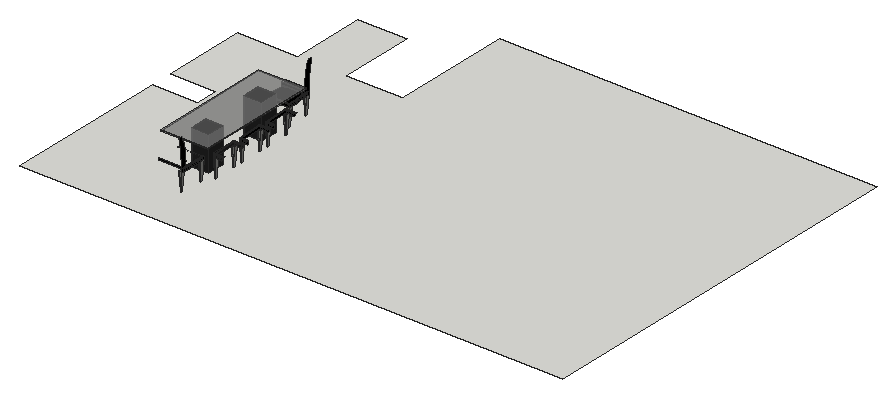
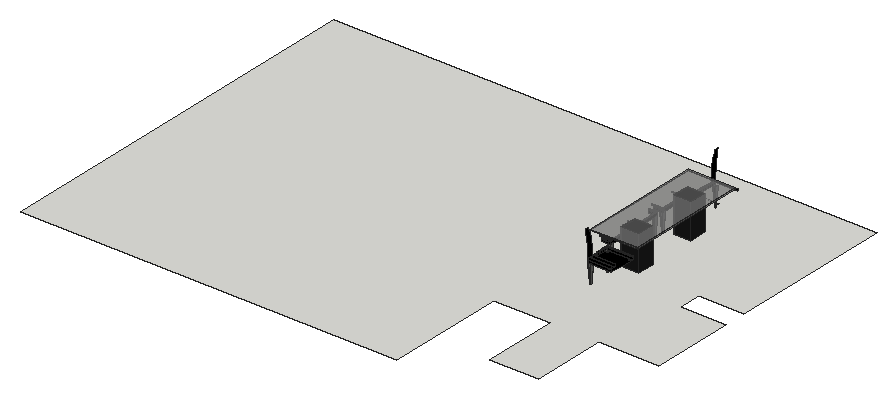
# SketchUp Ruby script. Lengths in inches.
U = 1.inch
M = Sketchup.active_model
def pt(a) = Geom::Point3d.new(a.map { |v| v * U })
def face(e, loops, mat)
  f = e.add_face(loops[0].map { |a| pt(a) })
  loops[1..].each { |l| e.add_face(l.map { |a| pt(a) }).erase! }
  f.material = f.back_material = mat if mat
  f
end
# faces: each face lists its corners as indices into pts; further lists are holes
def faces(e, pts, list, mat = nil) = list.each { |f| face(e, (f[0].is_a?(Array) ? f : [f]).map { |l| l.map { |i| pts[i] } }, mat) }
# xy, xz, yz: faces in a plane at the given z, y or x. An outline is a flat list of corners, or four numbers for a rectangle; further outlines are holes
def ring(l) = l.size == 4 ? [[l[0], l[1]], [l[2], l[1]], [l[2], l[3]], [l[0], l[3]]] : l.each_slice(2).to_a
def flat(e, list, mat, &to3) = list.each { |f| face(e, (f[0].is_a?(Array) ? f : [f]).map { |l| ring(l).map { |u, v| to3.(u, v) } }, mat) }
def xy(e, z, list, mat = nil) = flat(e, list, mat) { |x, y| [x, y, z] }
def xz(e, y, list, mat = nil) = flat(e, list, mat) { |x, z| [x, y, z] }
def yz(e, x, list, mat = nil) = flat(e, list, mat) { |y, z| [x, y, z] }
def lines(e, pts, list) = list.each { |a, b| e.add_line(pt(pts[a]), pt(pts[b])) }
# prism: a flat outline (further loops are holes) pulled along v
def prism(e, loops, v, mat = nil)
  f = face(e, loops, mat); d = Geom::Vector3d.new(v.map { |x| x * U })
  f.pushpull(f.normal.samedirection?(d) ? d.length : -d.length)
end
def box(e, o, s, mat = nil) = prism(e, [[o, [o[0] + s[0], o[1], o[2]], [o[0] + s[0], o[1] + s[1], o[2]], [o[0], o[1] + s[1], o[2]]]], [0, 0, s[2]], mat)
def at(x, y, z, deg = 0) = Geom::Transformation.translation(pt([x, y, z])) * Geom::Transformation.rotation(ORIGIN, Z_AXIS, deg.degrees)
def axes(o, x, y, z) = Geom::Transformation.new([*x, 0, *y, 0, *z, 0, *pt(o).to_a, 1])
def part(name) = M.definitions.add(name)
# library, detail: a bought-in or finely detailed component or shape, given as its bounding box
def library(name, o, s) = part(name).tap { |d| box(d.entities, o, s) }
def detail(e, o, s) = box(e.add_group.entities, o, s)
def put(e, d, t, mat = nil) = e.add_instance(d, t).tap { |i| i.material = mat if mat }
def group(e, t, mat = nil) = e.add_group.tap { |g| g.transformation = t; g.material = mat if mat }.entities
root = M.entities
M.materials.add("Color_008").color = [30, 30, 30]
M.materials.add("Translucent_Glass_Gray").color = [128, 128, 128]
M.materials["Translucent_Glass_Gray"].alpha = 0.5
M.materials.add("[Color M08]").color = [30, 30, 30]
M.materials.add("[Color M09]").color = [0, 0, 0]
M.materials.add("[Metal Seamed]").color = [118, 119, 115]
c1 = part("Dining table\#1")
xy(c1.entities,27.67,[[12.08,16.02,26.06,29.99],[12.08,68.04,26.06,82.01]],"Color_008")
xy(c1.entities,27.67,[[[0,0,38.14,98.03],[12.08,68.04,26.06,82.01],[12.08,16.02,26.06,29.99]]],"Translucent_Glass_Gray")
xy(c1.entities,28.85,[[0,0,38.14,98.03]],"Translucent_Glass_Gray")
xz(c1.entities,0,[[0,27.67,38.14,28.85]],"Translucent_Glass_Gray")
xz(c1.entities,16.02,[[12.08,0,26.06,27.67]],"Color_008")
xz(c1.entities,29.99,[[12.08,0,26.06,27.67]],"Color_008")
xz(c1.entities,68.04,[[12.08,0,26.06,27.67]],"Color_008")
xz(c1.entities,82.01,[[12.08,0,26.06,27.67]],"Color_008")
xz(c1.entities,98.03,[[0,27.67,38.14,28.85]],"Translucent_Glass_Gray")
yz(c1.entities,0,[[0,27.67,98.03,28.85]],"Translucent_Glass_Gray")
yz(c1.entities,12.08,[[16.02,0,29.99,27.67],[68.04,0,82.01,27.67]],"Color_008")
yz(c1.entities,26.06,[[16.02,0,29.99,27.67],[68.04,0,82.01,27.67]],"Color_008")
yz(c1.entities,38.14,[[0,27.67,98.03,28.85]],"Translucent_Glass_Gray")
xy(root,12,[[[24,24,456,24,456,336,156,336,156,240,110.625,240,110.625,300,72,300,72,240,24,240,24,174,60,174,60,156,24,156],[127.861,87.836,128.678,88.653],[146.137,88.857,146.954,89.674],[105.836,60.75,106.653,61.567],[146.137,114.763,146.954,115.58],[146.137,140.669,146.954,141.485],[81.769,105.091,82.586,105.908],[104.815,79.026,105.632,79.843],[127.861,113.742,128.678,114.558],[127.861,139.647,128.678,140.464],[81.769,156.903,82.586,157.72],[100.046,157.924,100.863,158.741],[81.769,130.997,82.586,131.814],[100.046,132.018,100.863,132.835],[100.046,106.112,100.863,106.929],[122.07,185.01,122.887,185.827],[123.092,166.733,123.908,167.55],[127.861,132.018,128.678,132.835],[146.137,105.091,146.954,105.908],[127.861,106.112,128.678,106.929],[122.07,60.75,122.887,61.567],[123.092,79.026,123.908,79.843],[146.137,130.997,146.954,131.814],[146.137,156.903,146.954,157.72],[81.769,140.669,82.586,141.485],[100.046,139.647,100.863,140.464],[81.769,88.857,82.586,89.674],[100.046,87.836,100.863,88.653],[105.836,185.01,106.653,185.827],[104.815,166.733,105.632,167.55],[81.769,114.763,82.586,115.58],[100.046,113.742,100.863,114.558],[127.861,157.924,128.678,158.741]]])
xy(root,12,[[122.07,60.75,122.887,61.567],[123.092,79.026,123.908,79.843],[127.861,87.836,128.678,88.653],[127.861,106.112,128.678,106.929],[127.861,113.742,128.678,114.558],
  [127.861,132.018,128.678,132.835],[127.861,139.647,128.678,140.464],[127.861,157.924,128.678,158.741],[123.092,166.733,123.908,167.55],[122.07,185.01,122.887,185.827]],"Color_008")
xy(root,26.704,[[121.406,60.085,123.552,62.231],[122.427,78.362,124.573,80.507],[127.197,87.171,129.342,89.317],[127.197,105.448,129.342,107.593],[127.197,113.077,129.342,115.223],
  [127.197,131.354,129.342,133.499],[127.197,138.983,129.342,141.129],[127.197,157.26,129.342,159.405],[122.427,166.069,124.573,168.214],[121.406,184.346,123.552,186.491]],"Color_008")
xy(root,26.704,[[104.151,166.069,104.08,167.774,104.038,169.481,104.024,171.1875,104.038,172.894,104.081,174.6,104.152,176.305,104.252,178.009,104.379,179.711,104.535,181.411,104.719,183.108,104.932,184.801,105.172,186.491,105.172,184.346,107.317,184.346,107.317,186.491,121.406,186.491,121.406,184.346,123.552,184.346,123.552,186.491,123.792,184.801,124.004,183.108,124.188,181.411,124.344,179.711,124.472,178.009,124.571,176.305,124.642,174.6,124.685,172.894,124.7,171.1875,124.686,169.481,124.643,167.774,124.573,166.069,124.573,168.214,122.427,168.214,122.427,166.069,106.296,166.069,106.296,168.214,104.151,168.214]],"[Color M09]")
xy(root,28.845,[[105.172,182.954,123.552,186.491]],"[Color M09]")
xz(root,166.069,[[104.151,26.704,124.573,28.845]],"[Color M09]")
xz(root,186.491,[[105.172,26.704,123.552,28.845]],"[Color M09]")
yz(root,123.552,[[60.085,28.845,60.059,30.792,59.999,32.738,59.905,34.683,59.777,36.626,59.615,38.566,59.419,40.503,59.189,42.436,58.925,44.365,58.628,46.29,58.297,48.208,57.932,50.121,57.534,52.027,59.985,52.027,60.713,50.191,61.367,48.328,61.945,46.44,62.446,44.53,62.87,42.602,63.216,40.658,63.482,38.701,63.67,36.736,63.777,34.764,63.806,32.79,63.754,30.816,63.622,28.845],[182.954,28.845,182.823,30.816,182.771,32.79,182.799,34.764,182.907,36.736,183.094,38.701,183.361,40.658,183.706,42.602,184.13,44.53,184.631,46.44,185.209,48.328,185.863,50.191,186.592,52.027,189.042,52.027,188.644,50.121,188.28,48.208,187.949,46.29,187.651,44.365,187.388,42.436,187.158,40.503,186.962,38.566,186.799,36.626,186.671,34.683,186.577,32.738,186.517,30.792,186.491,28.845]],"[Color M09]")
yz(root,127.197,[[87.171,26.704,107.593,28.845]],"[Color M08]")
yz(root,127.197,[[113.077,26.704,133.499,28.845],[138.983,26.704,159.405,28.845]],"[Color M09]")
p = [[121.406,62.231,26.704],[122.07,61.567,12],[122.07,60.75,12],[121.406,60.085,26.704],[122.887,60.75,12],[123.552,60.085,26.704],
  [122.887,61.567,12],[123.552,62.231,26.704],[122.427,80.507,26.704],[123.092,79.843,12],[123.092,79.026,12],[122.427,78.362,26.704],
  [123.908,79.026,12],[124.573,78.362,26.704],[123.908,79.843,12],[124.573,80.507,26.704],[127.197,89.317,26.704],[127.861,88.653,12],
  [127.861,87.836,12],[127.197,87.171,26.704],[128.678,87.836,12],[129.342,87.171,26.704],[128.678,88.653,12],[129.342,89.317,26.704],
  [127.861,106.112,12],[127.197,105.448,26.704],[127.197,107.593,26.704],[127.861,106.929,12],[128.678,106.112,12],[129.342,105.448,26.704],
  [128.678,106.929,12],[129.342,107.593,26.704],[127.197,115.223,26.704],[127.861,114.558,12],[127.861,113.742,12],[127.197,113.077,26.704],
  [128.678,113.742,12],[129.342,113.077,26.704],[128.678,114.558,12],[129.342,115.223,26.704],[127.861,132.018,12],[127.197,131.354,26.704],
  [127.197,133.499,26.704],[127.861,132.835,12],[128.678,132.018,12],[129.342,131.354,26.704],[128.678,132.835,12],[129.342,133.499,26.704],
  [127.197,141.129,26.704],[127.861,140.464,12],[127.861,139.647,12],[127.197,138.983,26.704],[128.678,139.647,12],[129.342,138.983,26.704],
  [128.678,140.464,12],[129.342,141.129,26.704],[127.861,157.924,12],[127.197,157.26,26.704],[127.197,159.405,26.704],[127.861,158.741,12],
  [128.678,157.924,12],[129.342,157.26,26.704],[128.678,158.741,12],[129.342,159.405,26.704],[123.092,166.733,12],[122.427,166.069,26.704],
  [122.427,168.214,26.704],[123.092,167.55,12],[123.908,166.733,12],[124.573,166.069,26.704],[123.908,167.55,12],[124.573,168.214,26.704],
  [122.07,185.01,12],[121.406,184.346,26.704],[121.406,186.491,26.704],[122.07,185.827,12],[122.887,185.01,12],[123.552,184.346,26.704],
  [122.887,185.827,12],[123.552,186.491,26.704],[123.792,61.775,26.704],[123.792,61.775,28.845],[123.552,60.085,28.845],[124.004,63.469,26.704],
  [124.004,63.469,28.845],[124.188,65.165,26.704],[124.188,65.165,28.845],[124.344,66.865,26.704],[124.344,66.865,28.845],[124.472,68.567,26.704],
  [124.472,68.567,28.845],[124.571,70.271,26.704],[124.571,70.271,28.845],[124.642,71.976,26.704],[124.642,71.976,28.845],[124.685,73.682,28.845],
  [124.685,73.682,26.704],[124.7,75.389,28.845],[124.7,75.389,26.704],[124.686,77.096,28.845],[124.686,77.096,26.704],[124.643,78.802,28.845],
  [124.643,78.802,26.704],[124.573,80.507,28.845],[132.315,87.045,28.845],[132.315,87.045,26.704],[130.608,87.058,26.704],[130.608,87.058,28.845],
  [134.022,87.059,28.845],[134.022,87.059,26.704],[128.902,87.101,28.845],[128.902,87.101,26.704],[127.197,87.171,28.845],[128.902,107.664,26.704],
  [128.902,107.664,28.845],[127.197,107.593,28.845],[130.608,107.706,26.704],[130.608,107.706,28.845],[132.315,107.72,26.704],[132.315,107.72,28.845],
  [134.022,107.706,26.704],[134.022,107.706,28.845],[128.902,113.007,28.845],[128.902,113.007,26.704],[127.197,113.077,28.845],[130.608,112.964,28.845],
  [130.608,112.964,26.704],[132.315,112.95,28.845],[132.315,112.95,26.704],[134.022,112.965,28.845],[134.022,112.965,26.704],[128.902,133.57,26.704],
  [128.902,133.57,28.845],[127.197,133.499,28.845],[130.608,133.612,26.704],[130.608,133.612,28.845],[132.315,133.626,26.704],[132.315,133.626,28.845],
  [134.022,133.612,26.704],[134.022,133.612,28.845],[128.902,138.913,28.845],[128.902,138.913,26.704],[127.197,138.983,28.845],[130.608,138.87,28.845],
  [130.608,138.87,26.704],[132.315,138.856,28.845],[132.315,138.856,26.704],[134.022,138.871,28.845],[134.022,138.871,26.704],[128.902,159.476,26.704],
  [128.902,159.476,28.845],[127.197,159.405,28.845],[130.608,159.518,26.704],[130.608,159.518,28.845],[132.315,159.532,26.704],[132.315,159.532,28.845],
  [134.022,159.517,26.704],[134.022,159.517,28.845],[124.643,167.774,28.845],[124.643,167.774,26.704],[124.573,166.069,28.845],[124.686,169.481,28.845],
  [124.686,169.481,26.704],[124.7,171.1875,28.845],[124.7,171.1875,26.704],[124.685,172.894,28.845],[124.685,172.894,26.704],[124.642,174.6,28.845],
  [124.642,174.6,26.704],[124.571,176.305,26.704],[124.571,176.305,28.845],[124.472,178.009,26.704],[124.472,178.009,28.845],[124.344,179.711,26.704],
  [124.344,179.711,28.845],[124.188,181.411,26.704],[124.188,181.411,28.845],[124.004,183.108,26.704],[124.004,183.108,28.845],[123.792,184.801,26.704],
  [123.792,184.801,28.845],[123.552,186.491,28.845],[105.172,60.085,28.845],[105.172,60.059,30.792],[123.552,60.059,30.792],[123.782,61.777,28.992],
  [123.543,60.095,28.992],[123.995,63.47,28.992],[124.179,65.166,28.992],[124.335,66.866,28.992],[124.462,68.568,28.992],[124.562,70.271,28.992],
  [124.633,71.976,28.992],[124.676,73.683,28.992],[124.69,75.389,28.992],[124.676,77.096,28.992],[124.634,78.802,28.992],[124.563,80.498,28.992],
  [104.16,80.498,28.992],[104.151,80.507,28.845],[132.315,87.054,28.992],[130.608,87.068,28.992],[134.021,87.069,28.992],[128.902,87.11,28.992],
  [127.206,87.181,28.992],[127.206,107.584,28.992],[128.902,107.654,28.992],[130.608,107.697,28.992],[132.315,107.71,28.992],[134.021,107.696,28.992],
  [128.902,113.016,28.992],[127.206,113.087,28.992],[130.608,112.974,28.992],[132.315,112.96,28.992],[134.021,112.974,28.992],[127.206,133.49,28.992],
  [128.902,133.56,28.992],[130.608,133.602,28.992],[132.315,133.616,28.992],[134.021,133.602,28.992],[128.902,138.922,28.992],[127.206,138.992,28.992],
  [130.608,138.88,28.992],[132.315,138.866,28.992],[134.021,138.88,28.992],[127.206,159.396,28.992],[128.902,159.466,28.992],[130.608,159.508,28.992],
  [132.315,159.522,28.992],[134.021,159.508,28.992],[124.563,166.079,28.992],[104.151,166.069,28.845],[104.16,166.079,28.992],[124.634,167.775,28.992],
  [124.676,169.481,28.992],[124.69,171.1875,28.992],[124.676,172.894,28.992],[124.633,174.6,28.992],[124.562,176.305,28.992],[124.462,178.009,28.992],
  [124.335,179.71,28.992],[124.179,181.41,28.992],[123.995,183.107,28.992],[123.552,182.823,30.816],[123.552,182.954,28.845],[105.172,182.954,28.845],
  [105.172,182.823,30.816],[123.782,184.8,28.992],[123.543,186.481,28.992],[123.552,186.517,30.792],[105.172,186.517,30.792],[105.172,186.491,28.845],
  [105.18,186.481,28.992],[123.754,61.78,29.137],[123.518,60.124,29.137],[123.966,63.473,29.137],[124.15,65.169,29.137],[124.306,66.868,29.137],
  [124.434,68.57,29.137],[124.533,70.273,29.137],[124.604,71.977,29.137],[124.647,73.683,29.137],[124.661,75.389,29.137],[124.647,77.095,29.137],
  [124.605,78.801,29.137],[124.536,80.469,29.137],[128.903,87.139,29.137],[127.235,87.208,29.137],[130.609,87.097,29.137],[132.315,87.083,29.137],
  [134.021,87.097,29.137],[127.235,107.556,29.137],[128.903,107.626,29.137],[130.609,107.668,29.137],[132.315,107.682,29.137],[134.021,107.667,29.137],
  [128.903,113.045,29.137],[127.235,113.114,29.137],[130.609,113.003,29.137],[132.315,112.989,29.137],[134.021,113.003,29.137],[127.235,133.462,29.137],
  [128.903,133.531,29.137],[130.609,133.574,29.137],[132.315,133.588,29.137],[134.021,133.573,29.137],[128.903,138.951,29.137],[127.235,139.02,29.137],
  [130.609,138.909,29.137],[132.315,138.895,29.137],[134.021,138.909,29.137],[127.235,159.368,29.137],[128.903,159.437,29.137],[130.609,159.48,29.137],
  [132.315,159.494,29.137],[134.021,159.479,29.137],[124.536,166.107,29.137],[104.188,166.107,29.137],[124.605,167.776,29.137],[124.647,169.481,29.137],
  [124.661,171.1875,29.137],[124.647,172.893,29.137],[124.604,174.599,29.137],[124.533,176.304,29.137],[124.434,178.007,29.137],[124.306,179.708,29.137],
  [124.15,181.407,29.137],[123.966,183.103,29.137],[123.754,184.796,29.137],[123.518,186.453,29.137],[105.205,186.453,29.137],[114.362,186.453,29.137],
  [123.477,60.171,29.276],[114.362,60.171,29.276],[114.362,60.124,29.137],[123.707,61.787,29.276],[123.919,63.479,29.276],[124.103,65.174,29.276],
  [124.259,66.872,29.276],[124.387,68.573,29.276],[124.486,70.275,29.276],[124.557,71.98,29.276],[124.557,71.978,29.276],[124.6,73.684,29.276],
  [124.614,75.389,29.276],[124.6,77.094,29.276],[124.558,78.799,29.276],[124.49,80.422,29.276],[128.905,87.186,29.276],[127.282,87.254,29.276],
  [130.61,87.144,29.276],[132.315,87.13,29.276],[134.02,87.145,29.276],[127.282,107.511,29.276],[128.905,107.578,29.276],[130.61,107.62,29.276],
  [132.315,107.634,29.276],[134.02,107.62,29.276],[128.905,113.092,29.276],[127.282,113.16,29.276],[130.61,113.05,29.276],[132.315,113.036,29.276],
  [134.02,113.05,29.276],[127.282,133.417,29.276],[128.905,133.484,29.276],[130.61,133.526,29.276],[132.315,133.54,29.276],[134.02,133.526,29.276],
  [130.61,138.956,29.276],[128.905,138.998,29.276],[132.315,138.942,29.276],[134.02,138.956,29.276],[127.282,139.065,29.276],[127.282,159.323,29.276],
  [128.905,159.39,29.276],[130.61,159.432,29.276],[132.315,159.446,29.276],[134.02,159.432,29.276],[124.49,166.155,29.276],[104.233,166.155,29.276],
  [124.558,167.777,29.276],[124.6,169.482,29.276],[124.614,171.1875,29.276],[124.6,172.893,29.276],[124.557,174.597,29.276],[124.486,176.301,29.276],
  [124.557,174.598,29.276],[124.387,178.004,29.276],[124.259,179.704,29.276],[124.103,181.402,29.276],[123.919,183.098,29.276],[123.707,184.79,29.276],
  [123.477,186.405,29.276],[114.362,186.405,29.276],[123.421,60.236,29.408],[114.362,60.236,29.408],[123.643,61.795,29.408],[123.855,63.486,29.408],
  [124.038,65.181,29.408],[124.194,66.878,29.408],[124.322,68.577,29.408],[124.421,70.278,29.408],[124.492,71.98,29.408],[124.492,71.982,29.408],
  [124.534,73.685,29.408],[124.549,75.389,29.408],[124.535,77.093,29.408],[124.493,78.797,29.408],[124.428,80.356,29.408],[130.611,87.209,29.408],
  [128.907,87.251,29.408],[132.315,87.195,29.408],[134.019,87.21,29.408],[127.347,87.316,29.408],[127.347,107.449,29.408],[128.907,107.513,29.408],
  [130.611,107.555,29.408],[132.315,107.569,29.408],[134.019,107.555,29.408],[132.315,113.101,29.408],[130.611,113.115,29.408],[134.019,113.116,29.408],
  [128.907,113.157,29.408],[127.347,113.222,29.408],[127.347,133.354,29.408],[128.907,133.419,29.408],[130.611,133.461,29.408],[132.315,133.475,29.408],
  [134.019,133.461,29.408],[132.315,139.007,29.408],[130.611,139.021,29.408],[134.019,139.021,29.408],[128.907,139.063,29.408],[127.347,139.128,29.408],
  [127.347,159.26,29.408],[128.907,159.325,29.408],[130.611,159.367,29.408],[132.315,159.381,29.408],[134.019,159.367,29.408],[124.428,166.22,29.408],
  [104.296,166.22,29.408],[124.493,167.779,29.408],[124.535,169.483,29.408],[124.549,171.1875,29.408],[124.534,172.891,29.408],[124.492,174.594,29.408],
  [124.421,176.298,29.408],[124.492,174.596,29.408],[124.322,177.999,29.408],[124.194,179.699,29.408],[124.038,181.396,29.408],[123.855,183.09,29.408],
  [123.643,184.781,29.408],[123.421,186.34,29.408],[114.362,186.34,29.408],[123.35,60.318,29.531],[114.362,60.318,29.531],[123.562,61.806,29.531],
  [123.773,63.496,29.531],[123.957,65.189,29.531],[124.113,66.884,29.531],[124.24,68.583,29.531],[124.339,70.283,29.531],[124.41,71.982,29.531],
  [124.41,71.986,29.531],[124.453,73.686,29.531],[124.467,75.389,29.531],[124.453,77.092,29.531],[124.411,78.794,29.531],[124.35,80.275,29.531],
  [130.612,87.291,29.531],[128.91,87.333,29.531],[132.315,87.277,29.531],[134.018,87.291,29.531],[127.429,87.395,29.531],[127.429,107.37,29.531],
  [128.91,107.431,29.531],[130.612,107.474,29.531],[132.315,107.488,29.531],[134.018,107.473,29.531],[130.612,113.197,29.531],[128.91,113.239,29.531],
  [132.315,113.183,29.531],[134.018,113.197,29.531],[127.429,113.3,29.531],[127.429,133.276,29.531],[128.91,133.337,29.531],[130.612,133.38,29.531],
  [132.315,133.393,29.531],[134.018,133.379,29.531],[130.612,139.103,29.531],[128.91,139.145,29.531],[132.315,139.089,29.531],[134.018,139.103,29.531],
  [127.429,139.206,29.531],[127.429,159.182,29.531],[128.91,159.243,29.531],[130.612,159.285,29.531],[132.315,159.299,29.531],[134.018,159.285,29.531],
  [124.35,166.302,29.531],[104.374,166.302,29.531],[124.411,167.782,29.531],[124.453,169.484,29.531],[124.467,171.1875,29.531],[124.453,172.89,29.531],
  [124.41,174.591,29.531],[124.339,176.294,29.531],[124.41,174.594,29.531],[124.24,177.994,29.531],[124.113,179.692,29.531],[123.957,181.388,29.531],
  [123.773,183.081,29.531],[123.562,184.77,29.531],[123.35,186.258,29.531],[114.362,186.258,29.531],[123.266,60.415,29.641],[114.362,60.415,29.641],
  [123.465,61.819,29.641],[123.677,63.507,29.641],[123.86,65.198,29.641],[124.016,66.892,29.641],[124.242,70.287,29.641],[124.143,68.589,29.641],
  [124.313,71.984,29.641],[124.313,71.99,29.641],[124.356,73.688,29.641],[124.37,75.389,29.641],[124.356,77.09,29.641],[124.314,78.791,29.641],
  [124.256,80.178,29.641],[128.913,87.43,29.641],[127.526,87.488,29.641],[130.614,87.388,29.641],[132.315,87.374,29.641],[134.016,87.388,29.641],
  [135.718,87.334,29.531],[135.714,87.431,29.641],[127.526,107.277,29.641],[128.913,107.334,29.641],[130.614,107.377,29.641],[135.718,107.431,29.531],
  [135.714,107.334,29.641],[134.016,107.376,29.641],[132.315,107.39,29.641],[128.913,139.242,29.641],[127.526,139.299,29.641],[130.614,139.2,29.641],
  [132.315,139.186,29.641],[134.016,139.2,29.641],[127.526,159.089,29.641],[128.913,159.146,29.641],[130.614,159.188,29.641],[135.718,159.242,29.531],
  [135.714,159.145,29.641],[134.016,159.188,29.641],[132.315,159.202,29.641],[123.677,183.069,29.641],[123.465,184.757,29.641],[123.266,186.161,29.641],
  [114.362,186.161,29.641]]
faces(root,p,[[0,1,2,3],[3,2,4,5],[6,7,5,4],[8,9,10,11],[11,10,12,13],[14,15,13,12],[9,8,15,14],[16,17,18,19],
  [19,18,20,21],[22,23,21,20],[17,16,23,22],[24,25,26,27],[25,24,28,29],[29,28,30,31],[27,26,31,30],[32,33,34,35],
  [35,34,36,37],[38,39,37,36],[33,32,39,38],[40,41,42,43],[41,40,44,45],[45,44,46,47],[43,42,47,46],[48,49,50,51],
  [51,50,52,53],[54,55,53,52],[49,48,55,54],[56,57,58,59],[61,60,62,63],[59,58,63,62],[64,65,66,67],[65,64,68,69],
  [69,68,70,71],[67,66,71,70],[72,73,74,75],[73,72,76,77],[77,76,78,79],[75,74,79,78]],"[Metal Seamed]")
faces(root,p,[[1,0,7,6],[57,56,60,61]],"Color_008")
faces(root,p,[[80,81,82,5],[83,84,81,80],[85,86,84,83],[87,88,86,85],[89,90,88,87],[91,92,90,89],[93,94,92,91],[93,94,95,96],
  [96,95,97,98],[98,97,99,100],[100,99,101,102],[102,101,103,15],[122,123,35,124],[125,126,123,122],[127,128,126,125],[129,130,128,127],
  [131,132,133,42],[134,135,132,131],[136,137,135,134],[138,139,137,136],[140,141,51,142],[143,144,141,140],[145,146,144,143],[147,148,146,145],
  [149,150,151,58],[152,153,150,149],[154,155,153,152],[156,157,155,154],[158,159,69,160],[161,162,159,158],[163,164,162,161],[165,166,164,163],
  [167,168,166,165],[167,168,169,170],[170,169,171,172],[172,171,173,174],[174,173,175,176],[176,175,177,178],[178,177,179,180],[180,179,79,181],
  [182,183,184,82],[81,185,186,82],[84,187,185,81],[86,188,187,84],[88,189,188,86],[90,190,189,88],[92,191,190,90],[94,192,191,92],
  [94,192,193,95],[95,193,194,97],[97,194,195,99],[99,195,196,101],[101,196,197,103],[198,199,103,197],[210,122,124,211],[212,125,122,210],
  [213,127,125,212],[214,129,127,213],[211,124,133,215],[132,216,215,133],[135,217,216,132],[137,218,217,135],[139,219,218,137],[220,140,142,221],
  [222,143,140,220],[223,145,143,222],[224,147,145,223],[221,142,151,225],[150,226,225,151],[153,227,226,150],[155,228,227,153],[157,229,228,155],
  [230,160,231,232],[233,158,160,230],[234,161,158,233],[235,163,161,234],[236,165,163,235],[237,167,165,236],[237,167,170,238],[238,170,172,239],
  [239,172,174,240],[240,174,176,241],[241,176,178,242],[243,244,245,246],[242,178,180,247],[247,180,181,248],[181,249,250,251],[248,181,251,252],
  [185,253,254,186],[187,255,253,185],[188,256,255,187],[189,257,256,188],[190,258,257,189],[191,259,258,190],[191,192,260,259],[192,260,261,193],
  [193,261,262,194],[194,262,263,195],[195,263,264,196],[196,264,265,197],[276,210,211,277],[278,212,210,276],[279,213,212,278],[280,214,213,279],
  [277,211,215,281],[216,282,281,215],[217,283,282,216],[218,284,283,217],[219,285,284,218],[286,220,221,287],[288,222,220,286],[289,223,222,288],
  [290,224,223,289],[287,221,225,291],[226,292,291,225],[227,293,292,226],[228,294,293,227],[229,295,294,228],[296,230,232,297],[298,233,230,296],
  [299,234,233,298],[300,235,234,299],[301,236,235,300],[302,237,236,301],[237,238,303,302],[303,238,239,304],[304,239,240,305],[305,240,241,306],
  [306,241,242,307],[307,242,247,308],[308,247,248,309],[309,248,252,310,311],[254,312,313,314],[253,315,312,254],[255,316,315,253],[256,317,316,255],
  [257,318,317,256],[258,319,318,257],[259,320,319,258],[260,321,322,320,259],[261,260,321,323],[261,323,324,262],[262,324,325,263],[263,325,326,264],
  [264,326,327,265],[338,276,277,339],[340,278,276,338],[341,279,278,340],[342,280,279,341],[339,277,281,343],[282,344,343,281],[283,345,344,282],
  [284,346,345,283],[285,347,346,284],[348,288,286,349],[350,289,288,348],[351,290,289,350],[352,287,291,353],[349,286,287,352],[292,354,353,291],
  [293,355,354,292],[294,356,355,293],[295,357,356,294],[358,296,297,359],[360,298,296,358],[361,299,298,360],[362,300,299,361],[363,301,300,362],
  [302,301,363,364],[364,302,303,365,366],[365,303,304,367],[367,304,305,368],[368,305,306,369],[369,306,307,370],[370,307,308,371],[371,308,309,372],
  [372,309,311,373],[312,374,375,313],[315,376,374,312],[316,377,376,315],[317,378,377,316],[318,379,378,317],[319,380,379,318],[320,381,380,319],
  [320,322,382,381],[382,383,321,322],[323,321,383,384],[323,384,385,324],[324,385,386,325],[325,386,387,326],[326,387,388,327],[399,341,340,400],
  [401,342,341,399],[402,338,339,403],[400,340,338,402],[403,339,343,404],[344,405,404,343],[345,406,405,344],[346,407,406,345],[347,408,407,346],
  [409,350,348,410],[411,351,350,409],[412,349,352,413],[410,348,349,412],[413,352,353,414],[354,415,414,353],[355,416,415,354],[356,417,416,355],
  [357,418,417,356],[419,358,359,420],[421,360,358,419],[422,361,360,421],[423,362,361,422],[424,363,362,423],[364,363,424,425],[366,365,426,427],
  [427,425,364,366],[426,365,367,428],[428,367,368,429],[429,368,369,430],[430,369,370,431],[431,370,371,432],[432,371,372,433],[433,372,373,434],
  [374,435,436,375],[376,437,435,374],[377,438,437,376],[378,439,438,377],[379,440,439,378],[380,441,440,379],[381,442,441,380],[381,382,443,442],
  [444,443,382,383],[384,383,444,445],[384,445,446,385],[385,446,447,386],[386,447,448,387],[387,448,449,388],[460,400,402,461],[462,399,400,460],
  [463,401,399,462],[464,403,404,465],[461,402,403,464],[405,466,465,404],[406,467,466,405],[407,468,467,406],[408,469,468,407],[470,410,412,471],
  [472,409,410,470],[473,411,409,472],[474,413,414,475],[471,412,413,474],[415,476,475,414],[416,477,476,415],[417,478,477,416],[418,479,478,417],
  [480,419,420,481],[482,421,419,480],[483,422,421,482],[484,423,422,483],[485,424,423,484],[425,424,485,486],[427,426,487,488],[486,488,427,425],
  [487,426,428,489],[489,428,429,490],[490,429,430,491],[491,430,431,492],[492,431,432,493],[493,432,433,494],[494,433,434,495],[435,496,497,436],
  [437,498,496,435],[438,499,498,437],[439,500,499,438],[440,501,500,439],[442,502,503,441],[442,443,504,502],[504,505,444,443],[445,506,507,446],
  [446,507,508,447],[447,508,509,448],[448,509,510,449],[525,471,474,526],[527,470,471,525],[528,472,470,527],[529,473,472,528],[526,474,475,530],
  [476,531,530,475],[477,532,531,476],[479,533,534,535],[478,536,532,477],[479,535,536,478],[537,492,493,538],[538,493,494,539],[539,494,495,540]],"[Color M09]")
faces(root,p,[[104,105,106,107],[108,109,105,104],[110,111,19,112],[107,106,111,110],[113,114,115,26],[116,117,114,113],[118,119,117,116],[120,121,119,118],
  [200,104,107,201],[202,108,104,200],[203,110,112,204],[201,107,110,203],[204,112,115,205],[114,206,205,115],[117,207,206,114],[119,208,207,117],
  [121,209,208,119],[266,203,204,267],[268,201,203,266],[269,200,201,268],[270,202,200,269],[267,204,205,271],[206,272,271,205],[207,273,272,206],
  [208,274,273,207],[209,275,274,208],[328,266,267,329],[330,268,266,328],[331,269,268,330],[332,270,269,331],[329,267,271,333],[272,334,333,271],
  [273,335,334,272],[274,336,335,273],[275,337,336,274],[389,330,328,390],[391,331,330,389],[392,332,331,391],[390,328,329,393],[393,329,333,394],
  [334,395,394,333],[335,396,395,334],[336,397,396,335],[337,398,397,336],[450,389,390,451],[452,391,389,450],[453,392,391,452],[454,393,394,455],
  [451,390,393,454],[395,456,455,394],[396,457,456,395],[397,458,457,396],[398,459,458,397],[511,451,454,512],[513,450,451,511],[514,452,450,513],
  [515,453,452,514],[516,453,515,517],[512,454,455,518],[456,519,518,455],[457,520,519,456],[459,521,522,523],[458,524,520,457],[459,523,524,458]],"[Color M08]")
put(root,c1,at(95.29,74.27,12))
